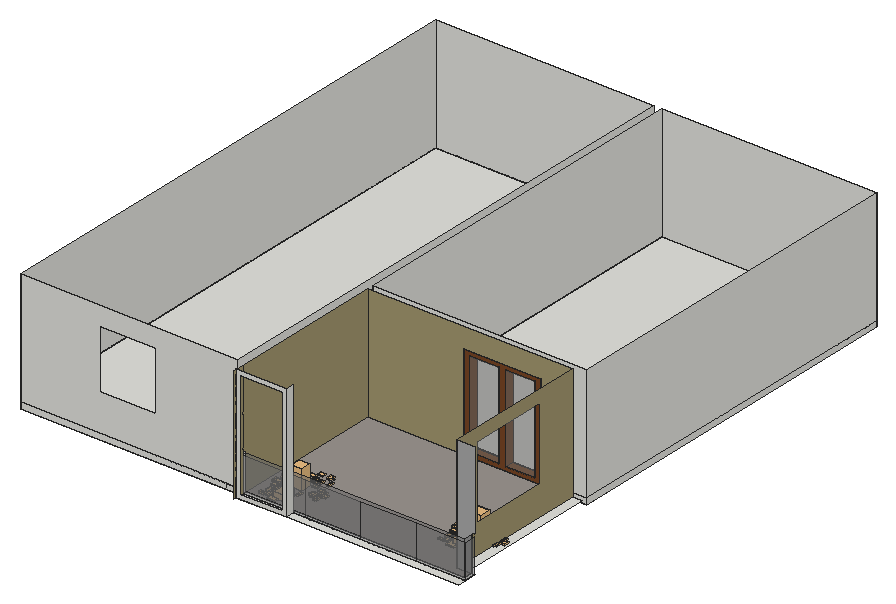
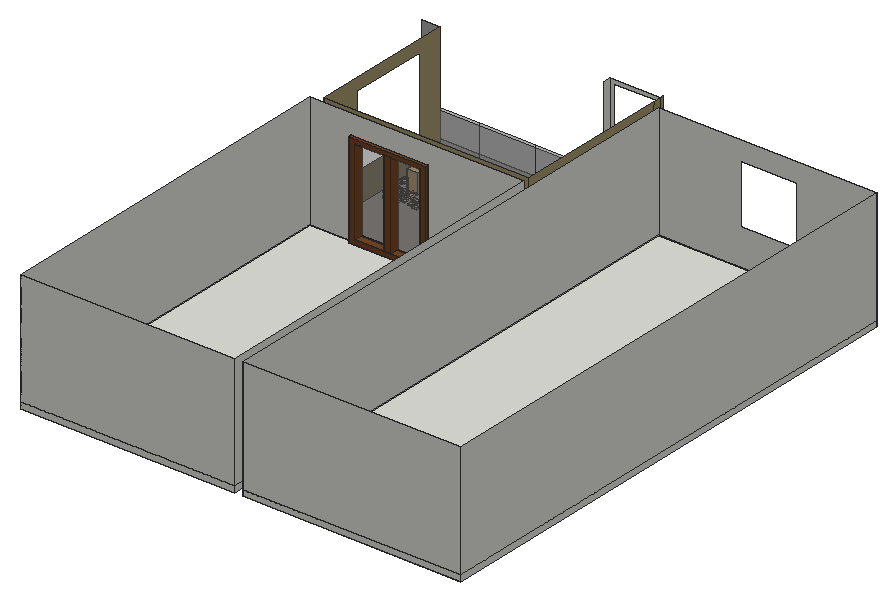
# SketchUp Ruby script. Lengths in inches.
U = 1.inch
M = Sketchup.active_model
def pt(a) = Geom::Point3d.new(a.map { |v| v * U })
def face(e, loops, mat)
  f = e.add_face(loops[0].map { |a| pt(a) })
  loops[1..].each { |l| e.add_face(l.map { |a| pt(a) }).erase! }
  f.material = f.back_material = mat if mat
  f
end
# faces: each face lists its corners as indices into pts; further lists are holes
def faces(e, pts, list, mat = nil) = list.each { |f| face(e, (f[0].is_a?(Array) ? f : [f]).map { |l| l.map { |i| pts[i] } }, mat) }
# xy, xz, yz: faces in a plane at the given z, y or x. An outline is a flat list of corners, or four numbers for a rectangle; further outlines are holes
def ring(l) = l.size == 4 ? [[l[0], l[1]], [l[2], l[1]], [l[2], l[3]], [l[0], l[3]]] : l.each_slice(2).to_a
def flat(e, list, mat, &to3) = list.each { |f| face(e, (f[0].is_a?(Array) ? f : [f]).map { |l| ring(l).map { |u, v| to3.(u, v) } }, mat) }
def xy(e, z, list, mat = nil) = flat(e, list, mat) { |x, y| [x, y, z] }
def xz(e, y, list, mat = nil) = flat(e, list, mat) { |x, z| [x, y, z] }
def yz(e, x, list, mat = nil) = flat(e, list, mat) { |y, z| [x, y, z] }
def lines(e, pts, list) = list.each { |a, b| e.add_line(pt(pts[a]), pt(pts[b])) }
# prism: a flat outline (further loops are holes) pulled along v
def prism(e, loops, v, mat = nil)
  f = face(e, loops, mat); d = Geom::Vector3d.new(v.map { |x| x * U })
  f.pushpull(f.normal.samedirection?(d) ? d.length : -d.length)
end
def box(e, o, s, mat = nil) = prism(e, [[o, [o[0] + s[0], o[1], o[2]], [o[0] + s[0], o[1] + s[1], o[2]], [o[0], o[1] + s[1], o[2]]]], [0, 0, s[2]], mat)
def at(x, y, z, deg = 0) = Geom::Transformation.translation(pt([x, y, z])) * Geom::Transformation.rotation(ORIGIN, Z_AXIS, deg.degrees)
def axes(o, x, y, z) = Geom::Transformation.new([*x, 0, *y, 0, *z, 0, *pt(o).to_a, 1])
def part(name) = M.definitions.add(name)
# library, detail: a bought-in or finely detailed component or shape, given as its bounding box
def library(name, o, s) = part(name).tap { |d| box(d.entities, o, s) }
def detail(e, o, s) = box(e.add_group.entities, o, s)
def put(e, d, t, mat = nil) = e.add_instance(d, t).tap { |i| i.material = mat if mat }
def group(e, t, mat = nil) = e.add_group.tap { |g| g.transformation = t; g.material = mat if mat }.entities
root = M.entities
M.materials.add("Bud_2").color = [160, 82, 113]
M.materials.add("Glass Realtime1").color = [156, 156, 156]
M.materials["Glass Realtime1"].alpha = 0.15
M.materials.add("Glass Red1").color = [0, 255, 255]
M.materials["Glass Red1"].alpha = 0.3
M.materials.add("Peony_Br1").color = [26, 30, 15]
M.materials.add("[Color M03]").color = [170, 170, 170]
M.materials.add("[Granite Tile]").color = [155, 148, 143]
M.materials.add("[Translucent Glass Gray]").color = [128, 128, 128]
M.materials["[Translucent Glass Gray]"].alpha = 0.5
M.materials.add("[Wood Lumber ButtJoined]").color = [164, 152, 112]
M.materials.add("[Wood Veneer 01]").color = [120, 70, 37]
c1 = part("Group\#1")
xy(c1.entities,0,[[0,0,48,9]],"[Wood Veneer 01]")
xy(c1.entities,3.71,[[3.71,0,21.93,9],[26.34,0,44.29,9]],"[Wood Veneer 01]")
xy(c1.entities,80.29,[[3.71,0,21.93,9],[26.34,0,44.29,9]],"[Wood Veneer 01]")
xy(c1.entities,84,[[0,0,48,9]],"[Wood Veneer 01]")
xz(c1.entities,0,[[3.71,3.71,21.93,80.29],[26.34,3.71,44.29,80.29]],"[Translucent Glass Gray]")
xz(c1.entities,0,[[[0,0,48,84],[3.71,3.71,21.93,80.29],[26.34,3.71,44.29,80.29]]],"[Wood Veneer 01]")
xz(c1.entities,9,[[[0,0,48,84],[3.71,3.71,44.29,80.29]],[21.93,3.71,26.34,80.29]],"[Wood Veneer 01]")
yz(c1.entities,0,[[0,0,9,84]],"[Wood Veneer 01]")
yz(c1.entities,3.71,[[0,3.71,9,80.29]],"[Wood Veneer 01]")
yz(c1.entities,21.93,[[0,3.71,9,80.29]],"[Wood Veneer 01]")
yz(c1.entities,26.34,[[0,3.71,9,80.29]],"[Wood Veneer 01]")
yz(c1.entities,44.29,[[0,3.71,9,80.29]],"[Wood Veneer 01]")
yz(c1.entities,48,[[0,0,9,84]],"[Wood Veneer 01]")
c2 = library("Group\#64",[-41.09,-203.71,-2.45],[72.23,68.1,8.96])
c3 = library("Group\#65",[-72.08,-328.41,-0.84],[78.06,90.26,14.33])
c4 = library("Group\#62",[-44.59,-71.91,-0.375],[108.06,108.06,265.92])
c5 = library("Group\#66",[-38.17,-273.34,-0.36],[93.61,85.68,37.86])
c6 = library("Group\#67",[-44.12,-281.8,-0.32],[111.26,106.83,75.57])
c7 = library("Group\#63",[-41.5,-68.73,2.45],[101.74,101.7,171.82])
xy(root,186,[[13.125,174.8125,241.5,718.875],[250.5,339.375,475.125,718.875]])
xy(root,192,[[250.5,161.01,303.24,169.32],[303.24,161.01,484.125,169.32],[250.5,169.32,250.5,173.51,480.43,173.51,480.43,182.19,484.125,182.19,484.125,169.32],[13.125,174.8125,241.5,718.875],[465.0625,182.19,475.125,333.375],
  [351.29,333.375,432.1,339.375],[250.5,339.375,475.125,718.875]])
xy(root,192,[[250.5,173.51,480.43,173.51,480.43,182.19,465.0625,182.19,465.0625,333.375,250.5,333.375]],"[Granite Tile]")
xz(root,161.01,[[[250.5,192,303.24,312.25],[254.52,196.02,299.22,308.23]]])
xz(root,169.32,[[250.5,192,303.24,228],[303.24,192,316.39,228],[316.39,192,374.26,228],[374.26,192,432.77,228],[432.77,192,484.125,228]],"[Translucent Glass Gray]")
xz(root,173.51,[[250.5,192,480.43,228]],"[Translucent Glass Gray]")
xz(root,174.8125,[[13.125,186,229,192],[229,186,241.5,192],[[13.125,192,241.5,312],[96.42,230.45,155.13,292.62]]])
xz(root,182.19,[[465.0625,192,480.43,192,480.43,230.3125,484.125,230.3125,484.125,312,465.0625,312]],"[Color M03]")
xz(root,333.375,[[250.5,192,351.29,192,351.29,291.4375,432.1,291.4375,432.1,192,465.0625,192,465.0625,312,250.5,312]],"[Wood Lumber ButtJoined]")
xz(root,339.375,[[250.5,186,351.29,192],[351.29,186,432.1,192],[432.1,186,445.8125,192],[445.8125,186,475.125,192],[250.5,192,250.5,312,475.125,312,475.125,192,432.1,192,432.1,291.4375,351.29,291.4375,351.29,192]])
xz(root,718.875,[[13.125,186,241.5,192],[250.5,186,475.125,192],[13.125,192,241.5,312],[250.5,192,475.125,312]])
yz(root,13.125,[[174.8125,186,718.875,192],[174.8125,192,718.875,312]])
yz(root,241.5,[[174.8125,186,718.875,192],[174.8125,192,718.875,312]])
yz(root,250.5,[[339.375,186,718.875,192],[169.32,192,173.51,228],[339.375,192,718.875,312]])
yz(root,250.5,[[157.82,192,161.01,312],[161.01,192,169.32,312],[173.51,192,333.375,192,333.375,312,169.32,312,169.32,230.3125,173.51,230.3125]],"[Wood Lumber ButtJoined]")
yz(root,303.24,[[161.01,192,169.32,312.25]])
yz(root,351.29,[[333.375,192,339.375,291.4375]])
yz(root,432.1,[[333.375,192,339.375,291.4375]])
yz(root,465.0625,[[[182.19,192,333.375,312],[207.39,223.41,290.14,299.35]]],"[Wood Lumber ButtJoined]")
yz(root,475.125,[[339.375,186,718.875,192],[339.375,192,718.875,312]])
yz(root,480.43,[[173.51,192,182.19,228]],"[Translucent Glass Gray]")
yz(root,484.125,[[169.32,192,182.19,228]],"[Translucent Glass Gray]")
p = [[279.06,209.92,192.1875],[279.16,209.92,192.1875],[279.16,210.03,192.1875],[441.92,241.33,192.1875],[442.03,241.33,192.1875],[442.03,241.44,192.1875]]
lines(root,p,[[0,1],[1,2],[2,0],[3,4],[4,5],[5,3]])
put(root,c1,axes([351.29,333.375,192],[1.68359,0,0],[0,1,0],[0,0,1.18378]))
put(root,c2,axes([279.06,209.92,192.1875],[0.1075,0,0],[0,0.1075,0],[0,0,0.0774]),"Peony_Br1")
put(root,c2,axes([441.92,241.33,192.1875],[0.1075,0,0],[0,0.1075,0],[0,0,0.0774]),"Peony_Br1")
g1 = group(root,at(279.06,209.92,192.1875),"Bud_2")
detail(g1,[-5.9,-14.63,-0.13],[5.36,2.04,0.85])
g2 = group(root,at(441.92,241.33,192.1875),"Bud_2")
detail(g2,[-5.9,-14.63,-0.13],[5.36,2.04,0.85])
g3 = group(root,at(279.06,209.92,192.1875),"Bud_2")
detail(g3,[20.81,-3.57,-0.13],[3.92,4.52,0.85])
g4 = group(root,at(441.92,241.33,192.1875),"Bud_2")
detail(g4,[20.81,-3.57,-0.13],[3.92,4.52,0.85])
g5 = group(root,at(279.06,209.92,192.1875),"Bud_2")
p = [[-13.21,22.51,0.21],[-13.11,22.36,0.08],[-13.21,23.11,-0.1],[-13.22,23.2,-0.04],[-15.51,18.89,0.15],[-14.6,19.57,0.01],
  [-13.87,20.48,0.33],[-15.4,18.86,-0.01],[-14.24,19.97,0.03],[-13.9,20.36,0.1],[-13.29,23.17,0.03],[-13.65,20.82,0.14],
  [-13.35,21.36,0.16],[-15.46,19.05,0.27],[-15.61,18.81,0.33],[-15.35,19.28,0.4],[-15.4,19.15,0.29],[-13.51,21.44,0.41],
  [-15.39,19.19,0.37],[-14.89,19.71,0.42],[-14.1,20.44,0.47],[-13.83,20.94,0.4375]]
faces(g5,p,[[0,1,2],[0,2,3],[4,5,6],[4,7,5],[8,6,5],[6,8,9],[3,10,0],[11,6,9],
  [6,11,12],[12,1,0],[4,13,14],[4,15,16],[13,4,16],[15,4,6],[6,12,17],[12,0,17],
  [15,18,16],[15,6,19],[6,20,19],[21,20,6],[6,17,21]],"Bud_2")
g6 = group(root,at(441.92,241.33,192.1875),"Bud_2")
p = [[-13.21,22.51,0.21],[-13.11,22.36,0.08],[-13.21,23.11,-0.1],[-13.22,23.2,-0.04],[-15.51,18.89,0.15],[-14.6,19.57,0.01],
  [-13.87,20.48,0.33],[-15.4,18.86,-0.01],[-14.24,19.97,0.03],[-13.9,20.36,0.1],[-13.29,23.17,0.03],[-13.65,20.82,0.14],
  [-13.35,21.36,0.16],[-15.46,19.05,0.27],[-15.61,18.81,0.33],[-15.35,19.28,0.4],[-15.4,19.15,0.29],[-13.51,21.44,0.41],
  [-15.39,19.19,0.37],[-14.89,19.71,0.42],[-14.1,20.44,0.47],[-13.83,20.94,0.4375]]
faces(g6,p,[[0,1,2],[0,2,3],[4,5,6],[4,7,5],[8,6,5],[6,8,9],[3,10,0],[11,6,9],
  [6,11,12],[12,1,0],[4,13,14],[4,15,16],[13,4,16],[15,4,6],[6,12,17],[12,0,17],
  [15,18,16],[15,6,19],[6,20,19],[21,20,6],[6,17,21]],"Bud_2")
g7 = group(root,at(279.06,209.92,192.1875),"Bud_2")
detail(g7,[2.23,12.49,-0.1],[2.04,5.3,0.86])
g8 = group(root,at(441.92,241.33,192.1875),"Bud_2")
detail(g8,[2.23,12.49,-0.1],[2.04,5.3,0.86])
g9 = group(root,at(279.06,209.92,192.1875),"Bud_2")
detail(g9,[-4.74,16.83,-0.09],[4.84,3.9,0.78])
g10 = group(root,at(441.92,241.33,192.1875),"Bud_2")
detail(g10,[-4.74,16.83,-0.09],[4.84,3.9,0.78])
g11 = group(root,at(279.06,209.92,192.1875),"Bud_2")
p = [[9.02,9.01,-0.02],[9.69,8.43,0],[9.61,8.46,-0.08],[8.9,9.11,0.18],[9.6,8.42,0.07],[7.97,9.7,0.3125],
  [7.95,9.77,0.01],[6.82,10.16,0.23],[7.27,9.95,0.02],[6.65,10.18,0.03],[4.65,10.31,-0.01],[4.16,10.26,0.24],
  [5.39,10.26,0.01],[4.48,10.27,0.1],[4.54,10.32,0.02],[4.35,10.29,0.13],[4.18,10.38,0.05],[7.27,9.87,0.37],
  [6.68,10.03,0.45],[6.07,10.0625,0.5],[5.45,10.14,0.5],[4.22,10.21,0.43]]
faces(g11,p,[[0,1,2],[0,3,4],[0,4,1],[5,0,6],[5,3,0],[7,5,6],[7,6,8],[8,9,7],
  [10,11,7],[10,7,12],[7,9,12],[11,10,13],[13,10,14],[11,15,16],[15,11,13],[7,17,5],
  [17,7,18],[7,19,18],[11,20,7],[11,21,20],[19,7,20]],"Bud_2")
g12 = group(root,at(441.92,241.33,192.1875),"Bud_2")
p = [[9.02,9.01,-0.02],[9.69,8.43,0],[9.61,8.46,-0.08],[8.9,9.11,0.18],[9.6,8.42,0.07],[7.97,9.7,0.3125],
  [7.95,9.77,0.01],[6.82,10.16,0.23],[7.27,9.95,0.02],[6.65,10.18,0.03],[4.65,10.31,-0.01],[4.16,10.26,0.24],
  [5.39,10.26,0.01],[4.48,10.27,0.1],[4.54,10.32,0.02],[4.35,10.29,0.13],[4.18,10.38,0.05],[7.27,9.87,0.37],
  [6.68,10.03,0.45],[6.07,10.0625,0.5],[5.45,10.14,0.5],[4.22,10.21,0.43]]
faces(g12,p,[[0,1,2],[0,3,4],[0,4,1],[5,0,6],[5,3,0],[7,5,6],[7,6,8],[8,9,7],
  [10,11,7],[10,7,12],[7,9,12],[11,10,13],[13,10,14],[11,15,16],[15,11,13],[7,17,5],
  [17,7,18],[7,19,18],[11,20,7],[11,21,20],[19,7,20]],"Bud_2")
g13 = group(root,at(279.06,209.92,192.1875),"Bud_2")
detail(g13,[-22.32,3.27,-0.07],[2.75,5.4,0.95])
g14 = group(root,at(441.92,241.33,192.1875),"Bud_2")
detail(g14,[-22.32,3.27,-0.07],[2.75,5.4,0.95])
g15 = group(root,at(279.06,209.92,192.1875),"Bud_2")
p = [[-7.58,-14.37,0.05],[-7.375,-14.31,-0.07],[-7.1,-13.11,0.05],[-7.67,-8.62,-0.0625],[-7.74,-8.53,-0.01],[-7.4375,-9.36,0.1],
  [-7.55,-9.5625,0.28],[-7.83,-8.61,0.04],[-7.77,-13.9,0.29],[-7.6875,-14.06,0.1875],[-7.15,-11.79,0.43],[-7.67,-14.1875,0.16],
  [-7.75,-14.37,0.23],[-7.02,-12.5,0.11],[-6.99,-11.9,0.22],[-7.39,-10.58,0.5],[-7.06,-10.58,0.3],[-7.75,-14.01,0.26],
  [-7.04,-11.29,0.26],[-7.63,-13.17,0.375],[-7.4,-11.95,0.52],[-7.42,-11.29,0.49]]
faces(g15,p,[[0,1,2],[3,4,5],[6,4,7],[6,5,4],[0,8,9],[8,0,10],[0,11,12],[11,0,9],
  [0,2,10],[13,10,2],[10,13,14],[15,5,6],[15,16,5],[9,8,17],[18,10,14],[8,10,19],
  [10,16,15],[10,18,16],[10,20,19],[10,21,20],[10,15,21]],"Bud_2")
g16 = group(root,at(441.92,241.33,192.1875),"Bud_2")
p = [[-7.58,-14.37,0.05],[-7.375,-14.31,-0.07],[-7.1,-13.11,0.05],[-7.67,-8.62,-0.0625],[-7.74,-8.53,-0.01],[-7.4375,-9.36,0.1],
  [-7.55,-9.5625,0.28],[-7.83,-8.61,0.04],[-7.77,-13.9,0.29],[-7.6875,-14.06,0.1875],[-7.15,-11.79,0.43],[-7.67,-14.1875,0.16],
  [-7.75,-14.37,0.23],[-7.02,-12.5,0.11],[-6.99,-11.9,0.22],[-7.39,-10.58,0.5],[-7.06,-10.58,0.3],[-7.75,-14.01,0.26],
  [-7.04,-11.29,0.26],[-7.63,-13.17,0.375],[-7.4,-11.95,0.52],[-7.42,-11.29,0.49]]
faces(g16,p,[[0,1,2],[3,4,5],[6,4,7],[6,5,4],[0,8,9],[8,0,10],[0,11,12],[11,0,9],
  [0,2,10],[13,10,2],[10,13,14],[15,5,6],[15,16,5],[9,8,17],[18,10,14],[8,10,19],
  [10,16,15],[10,18,16],[10,20,19],[10,21,20],[10,15,21]],"Bud_2")
g17 = group(root,at(279.06,209.92,192.1875),"Bud_2")
p = [[21.18,-5.17,0.05],[21.23,-4.96,-0.07],[20.34,-4.12,0.05],[16.16,-2.37,-0.0625],[16.05,-2.39,-0.01],[16.91,-2.54,0.1],
  [17.03,-2.74,0.28],[16.07,-2.5,0.04],[20.98,-5.16,0.16],[21.1,-5.3125,0.23],[19.17,-3.51,0.43],[20.68,-5.1,0.29],
  [20.86,-5.11,0.1875],[19.84,-3.75,0.11],[19.34,-3.42,0.22],[18,-3.11,0.5],[18.16,-2.83,0.3],[20.79,-5.13,0.26],
  [18.78,-3.16,0.26],[20.12,-4.62,0.375],[19.18,-3.81,0.52],[18.6,-3.49,0.49]]
faces(g17,p,[[0,1,2],[3,4,5],[6,4,7],[6,5,4],[0,8,9],[0,2,10],[11,0,10],[0,11,12],
  [8,0,12],[13,10,2],[10,13,14],[15,5,6],[15,16,5],[12,11,17],[18,10,14],[11,10,19],
  [10,16,15],[10,18,16],[10,20,19],[10,21,20],[10,15,21]],"Bud_2")
g18 = group(root,at(441.92,241.33,192.1875),"Bud_2")
p = [[21.18,-5.17,0.05],[21.23,-4.96,-0.07],[20.34,-4.12,0.05],[16.16,-2.37,-0.0625],[16.05,-2.39,-0.01],[16.91,-2.54,0.1],
  [17.03,-2.74,0.28],[16.07,-2.5,0.04],[20.98,-5.16,0.16],[21.1,-5.3125,0.23],[19.17,-3.51,0.43],[20.68,-5.1,0.29],
  [20.86,-5.11,0.1875],[19.84,-3.75,0.11],[19.34,-3.42,0.22],[18,-3.11,0.5],[18.16,-2.83,0.3],[20.79,-5.13,0.26],
  [18.78,-3.16,0.26],[20.12,-4.62,0.375],[19.18,-3.81,0.52],[18.6,-3.49,0.49]]
faces(g18,p,[[0,1,2],[3,4,5],[6,4,7],[6,5,4],[0,8,9],[0,2,10],[11,0,10],[0,11,12],
  [8,0,12],[13,10,2],[10,13,14],[15,5,6],[15,16,5],[12,11,17],[18,10,14],[11,10,19],
  [10,16,15],[10,18,16],[10,20,19],[10,21,20],[10,15,21]],"Bud_2")
put(root,c3,axes([279.06,209.92,192.1875],[0.1075,0,0],[0,0.1075,0],[0,0,0.0774]),"Peony_Br1")
put(root,c3,axes([441.92,241.33,192.1875],[0.1075,0,0],[0,0.1075,0],[0,0,0.0774]),"Peony_Br1")
g19 = group(root,at(279.06,209.92,192.1875),"Bud_2")
detail(g19,[-11.87,10.35,-0.0625],[4.93,4.51,0.74])
g20 = group(root,at(441.92,241.33,192.1875),"Bud_2")
detail(g20,[-11.87,10.35,-0.0625],[4.93,4.51,0.74])
g21 = group(root,at(279.06,209.92,192.1875),"Bud_2")
detail(g21,[-2.95,-13.39,-0.06],[2.25,5.14,0.71])
g22 = group(root,at(441.92,241.33,192.1875),"Bud_2")
detail(g22,[-2.95,-13.39,-0.06],[2.25,5.14,0.71])
g23 = group(root,at(279.06,209.92,192.1875),"Bud_2")
detail(g23,[17.98,-11.125,-0.05],[6.2,2.875,0.8])
g24 = group(root,at(441.92,241.33,192.1875),"Bud_2")
detail(g24,[17.98,-11.125,-0.05],[6.2,2.875,0.8])
g25 = group(root,at(279.06,209.92,192.1875),"Bud_2")
detail(g25,[-21.5,-9.1,-0.05],[6.35,4.98,1])
g26 = group(root,at(441.92,241.33,192.1875),"Bud_2")
detail(g26,[-21.5,-9.1,-0.05],[6.35,4.98,1])
g27 = group(root,at(279.06,209.92,192.1875),"Bud_2")
p = [[11.24,21.1,0.17],[12.16,22.02,-0.04],[13.25,22.87,0.28],[11.25,21.19,-0.01],[12.66,22.4,-0.03],[13.14,22.77,0.03],
  [13.71,23.03,0.08],[15.65,23.34,0.23],[15.47,23.45,0.08],[16.44,23.32,-0.03],[16.54,23.33,0.05],[14.35,23.34,0.11],
  [14.39,23.24,0.4],[16.48,23.28,0.12],[11.64,21.34,0.44],[11.51,21.26,0.32],[11.39,21.19,0.3],[11.24,21.1,0.38],
  [11.54,21.29,0.41],[12.21,21.83,0.44],[13.16,22.66,0.45],[13.77,22.91,0.43]]
faces(g27,p,[[0,1,2],[0,3,1],[4,2,1],[2,4,5],[6,2,5],[7,8,9],[7,9,10],[2,11,12],
  [2,6,11],[7,12,11],[7,11,8],[10,13,7],[0,14,15],[0,16,17],[16,0,15],[14,0,2],
  [15,14,18],[14,2,19],[2,20,19],[2,21,20],[12,21,2]],"Bud_2")
g28 = group(root,at(441.92,241.33,192.1875),"Bud_2")
p = [[11.24,21.1,0.17],[12.16,22.02,-0.04],[13.25,22.87,0.28],[11.25,21.19,-0.01],[12.66,22.4,-0.03],[13.14,22.77,0.03],
  [13.71,23.03,0.08],[15.65,23.34,0.23],[15.47,23.45,0.08],[16.44,23.32,-0.03],[16.54,23.33,0.05],[14.35,23.34,0.11],
  [14.39,23.24,0.4],[16.48,23.28,0.12],[11.64,21.34,0.44],[11.51,21.26,0.32],[11.39,21.19,0.3],[11.24,21.1,0.38],
  [11.54,21.29,0.41],[12.21,21.83,0.44],[13.16,22.66,0.45],[13.77,22.91,0.43]]
faces(g28,p,[[0,1,2],[0,3,1],[4,2,1],[2,4,5],[6,2,5],[7,8,9],[7,9,10],[2,11,12],
  [2,6,11],[7,12,11],[7,11,8],[10,13,7],[0,14,15],[0,16,17],[16,0,15],[14,0,2],
  [15,14,18],[14,2,19],[2,20,19],[2,21,20],[12,21,2]],"Bud_2")
g29 = group(root,at(279.06,209.92,192.1875),"Bud_2")
p = [[-8.66,14.35,0.55],[-8.67,14.46,0.49],[-10.8,15.02,-0.04],[-9.67,14.46,0.32],[-10.64,14.57,0.1],[-11.17,14.86,0],
  [-11.24,14.67,0.15],[-12.08,15.08,0.3],[-11.54,15.1875,0.16],[-13.82,15.57,0.05],[-13.57,15.88,0.04],[-13.74,16.03,0.03],
  [-13.43,15.85,0.0625],[-13.125,15.27,0.26],[-13.33,15.94,0.08],[-12.49,15.56,0.22],[-11.73,14.73,0.31],[-11.95,15.36,0.3],
  [-8.78,14.28,0.59],[-12.2,14.82,0.43],[-12.69,14.97,0.33]]
faces(g29,p,[[0,1,2],[2,3,0],[3,2,4],[5,4,2],[5,6,4],[7,6,5],[7,5,2],[7,2,8],
  [9,10,11],[9,12,10],[7,12,9],[13,7,9],[7,14,12],[7,15,14],[7,16,6],[7,17,15],
  [8,17,7],[18,0,3],[16,7,19],[7,20,19],[7,13,20]],"Bud_2")
g30 = group(root,at(441.92,241.33,192.1875),"Bud_2")
p = [[-8.66,14.35,0.55],[-8.67,14.46,0.49],[-10.8,15.02,-0.04],[-9.67,14.46,0.32],[-10.64,14.57,0.1],[-11.17,14.86,0],
  [-11.24,14.67,0.15],[-12.08,15.08,0.3],[-11.54,15.1875,0.16],[-13.82,15.57,0.05],[-13.57,15.88,0.04],[-13.74,16.03,0.03],
  [-13.43,15.85,0.0625],[-13.125,15.27,0.26],[-13.33,15.94,0.08],[-12.49,15.56,0.22],[-11.73,14.73,0.31],[-11.95,15.36,0.3],
  [-8.78,14.28,0.59],[-12.2,14.82,0.43],[-12.69,14.97,0.33]]
faces(g30,p,[[0,1,2],[2,3,0],[3,2,4],[5,4,2],[5,6,4],[7,6,5],[7,5,2],[7,2,8],
  [9,10,11],[9,12,10],[7,12,9],[13,7,9],[7,14,12],[7,15,14],[7,16,6],[7,17,15],
  [8,17,7],[18,0,3],[16,7,19],[7,20,19],[7,13,20]],"Bud_2")
g31 = group(root,at(279.06,209.92,192.1875),"Bud_2")
detail(g31,[-18.57,4.34,-0.04],[2.34,4.87,1.26])
g32 = group(root,at(441.92,241.33,192.1875),"Bud_2")
detail(g32,[-18.57,4.34,-0.04],[2.34,4.87,1.26])
g33 = group(root,at(279.06,209.92,192.1875),"Bud_2")
detail(g33,[-13.99,0.47,-0.04],[5.21,5.59,0.87])
g34 = group(root,at(441.92,241.33,192.1875),"Bud_2")
detail(g34,[-13.99,0.47,-0.04],[5.21,5.59,0.87])
g35 = group(root,at(279.06,209.92,192.1875),"Bud_2")
detail(g35,[-21.22,10.73,-0.04],[4.63,4.04,1.21])
g36 = group(root,at(441.92,241.33,192.1875),"Bud_2")
detail(g36,[-21.22,10.73,-0.04],[4.63,4.04,1.21])
g37 = group(root,at(279.06,209.92,192.1875),"Bud_2")
detail(g37,[17.42,0.48,-0.03],[4.12,3.84,0.71])
g38 = group(root,at(441.92,241.33,192.1875),"Bud_2")
detail(g38,[17.42,0.48,-0.03],[4.12,3.84,0.71])
g39 = group(root,at(279.06,209.92,192.1875),"Bud_2")
detail(g39,[7.79,-15.84,-0.03],[2.5,5.05,0.71])
g40 = group(root,at(441.92,241.33,192.1875),"Bud_2")
detail(g40,[7.79,-15.84,-0.03],[2.5,5.05,0.71])
g41 = group(root,at(279.06,209.92,192.1875),"Bud_2")
detail(g41,[-16.14,-25.87,-0.03],[1.25,5.39,1.93])
g42 = group(root,at(441.92,241.33,192.1875),"Bud_2")
detail(g42,[-16.14,-25.87,-0.03],[1.25,5.39,1.93])
g43 = group(root,at(279.06,209.92,192.1875),"Bud_2")
detail(g43,[-18.74,-31.57,-0.03],[5.12,2.12,1.39])
g44 = group(root,at(441.92,241.33,192.1875),"Bud_2")
detail(g44,[-18.74,-31.57,-0.03],[5.12,2.12,1.39])
put(root,c4,axes([279.06,209.92,192.1875],[0.1075,0,0],[0,0.1075,0],[0,0,0.0774]),"Glass Realtime1")
put(root,c4,axes([441.92,241.33,192.1875],[0.1075,0,0],[0,0.1075,0],[0,0,0.0774]),"Glass Realtime1")
put(root,c5,axes([279.06,209.92,192.1875],[0.1075,0,0],[0,0.1075,0],[0,0,0.0774]),"Peony_Br1")
put(root,c5,axes([441.92,241.33,192.1875],[0.1075,0,0],[0,0.1075,0],[0,0,0.0774]),"Peony_Br1")
g45 = group(root,at(279.06,209.92,192.1875),"Bud_2")
p = [[-4.24,-9.44,0.05],[-4.38,-10.24,0.125],[-4.45,-10.28,0.05],[-4.41,-10.21,-0.03],[-4.16,-9.26,0.25],[-3.78,-8.2,0.1],
  [-3.73,-8.28,0.39],[-2.99,-7.32,0.3],[-2.83,-7.2,0.1],[-1.74,-6.58,0.03],[-1.1,-6.2,-0.01],[-0.625,-6.03,0.23],
  [-0.92,-6.16,0.1],[-1,-6.14,0.02],[-0.82,-6.09,0.12],[-0.71,-5.93,0.04],[-3.27,-7.7,0.09],[-1.7,-6.72,0.52],
  [-0.64,-6.12,0.41],[-3.21,-7.78,0.44],[-2.76,-7.37,0.51],[-2.22,-7.07,0.54]]
faces(g45,p,[[0,1,2],[2,3,0],[0,4,1],[5,6,0],[6,4,0],[7,8,9],[10,7,9],[10,11,7],
  [11,10,12],[12,10,13],[11,14,15],[7,6,5],[7,5,16],[7,16,8],[14,11,12],[11,17,7],
  [11,18,17],[7,19,6],[19,7,20],[7,21,20],[21,7,17]],"Bud_2")
g46 = group(root,at(441.92,241.33,192.1875),"Bud_2")
p = [[-4.24,-9.44,0.05],[-4.38,-10.24,0.125],[-4.45,-10.28,0.05],[-4.41,-10.21,-0.03],[-4.16,-9.26,0.25],[-3.78,-8.2,0.1],
  [-3.73,-8.28,0.39],[-2.99,-7.32,0.3],[-2.83,-7.2,0.1],[-1.74,-6.58,0.03],[-1.1,-6.2,-0.01],[-0.625,-6.03,0.23],
  [-0.92,-6.16,0.1],[-1,-6.14,0.02],[-0.82,-6.09,0.12],[-0.71,-5.93,0.04],[-3.27,-7.7,0.09],[-1.7,-6.72,0.52],
  [-0.64,-6.12,0.41],[-3.21,-7.78,0.44],[-2.76,-7.37,0.51],[-2.22,-7.07,0.54]]
faces(g46,p,[[0,1,2],[2,3,0],[0,4,1],[5,6,0],[6,4,0],[7,8,9],[10,7,9],[10,11,7],
  [11,10,12],[12,10,13],[11,14,15],[7,6,5],[7,5,16],[7,16,8],[14,11,12],[11,17,7],
  [11,18,17],[7,19,6],[19,7,20],[7,21,20],[21,7,17]],"Bud_2")
put(root,c6,axes([279.06,209.92,192.1875],[0.1075,0,0],[0,0.1075,0],[0,0,0.0774]),"Bud_2")
put(root,c6,axes([441.92,241.33,192.1875],[0.1075,0,0],[0,0.1075,0],[0,0,0.0774]),"Bud_2")
g47 = group(root,at(279.06,209.92,192.1875),"Bud_2")
detail(g47,[-24.68,16.18,-0.02],[5.31,2.02,0.74])
g48 = group(root,at(441.92,241.33,192.1875),"Bud_2")
detail(g48,[-24.68,16.18,-0.02],[5.31,2.02,0.74])
g49 = group(root,at(279.06,209.92,192.1875),"Bud_2")
detail(g49,[-13.74,-19.43,-0.02],[3.5,5.54,0.81])
g50 = group(root,at(441.92,241.33,192.1875),"Bud_2")
detail(g50,[-13.74,-19.43,-0.02],[3.5,5.54,0.81])
g51 = group(root,at(279.06,209.92,192.1875),"Bud_2")
detail(g51,[22.58,-3.19,-0.02],[4.21,5.66,1.15])
g52 = group(root,at(441.92,241.33,192.1875),"Bud_2")
detail(g52,[22.58,-3.19,-0.02],[4.21,5.66,1.15])
g53 = group(root,at(279.06,209.92,192.1875),"Bud_2")
detail(g53,[-13.66,-30.82,-0.01],[3.6,5.41,0.92])
g54 = group(root,at(441.92,241.33,192.1875),"Bud_2")
detail(g54,[-13.66,-30.82,-0.01],[3.6,5.41,0.92])
g55 = group(root,at(279.06,209.92,192.1875),"Bud_2")
detail(g55,[-19.59,-15.02,-0.01],[6.1,4.3,1.1])
g56 = group(root,at(441.92,241.33,192.1875),"Bud_2")
detail(g56,[-19.59,-15.02,-0.01],[6.1,4.3,1.1])
g57 = group(root,at(279.06,209.92,192.1875),"Bud_2")
detail(g57,[-22.52,-9.47,-0.01],[1.45,5.49,1.23])
g58 = group(root,at(441.92,241.33,192.1875),"Bud_2")
detail(g58,[-22.52,-9.47,-0.01],[1.45,5.49,1.23])
g59 = group(root,at(279.06,209.92,192.1875),"Bud_2")
detail(g59,[26.73,-5.87,-0.01],[3.91,4.56,1.35])
g60 = group(root,at(441.92,241.33,192.1875),"Bud_2")
detail(g60,[26.73,-5.87,-0.01],[3.91,4.56,1.35])
g61 = group(root,at(279.06,209.92,192.1875),"Bud_2")
detail(g61,[-19.41,20.4,0],[5.31,3.52,1.58])
g62 = group(root,at(441.92,241.33,192.1875),"Bud_2")
detail(g62,[-19.41,20.4,0],[5.31,3.52,1.58])
g63 = group(root,at(279.06,209.92,192.1875),"Bud_2")
detail(g63,[-4.3,7.33,0],[4.16,5.19,2.05])
g64 = group(root,at(441.92,241.33,192.1875),"Bud_2")
detail(g64,[-4.3,7.33,0],[4.16,5.19,2.05])
g65 = group(root,at(279.06,209.92,192.1875),"Bud_2")
p = [[-10.97,-5.54,0.2],[-10.36,-6.01,0.01],[-10.41,-6.15,0.03],[-10.51,-6.13,0.01],[-10.83,-5.31,0.28],[-12.14,-3.64,0.17],
  [-12.32,-3.27,0],[-12.11,-3.07,0.08],[-12.6875,-2.8125,0.02],[-11.71,-3.33,0.17],[-11.85,-2.88,0.04],[-13.33,-2.11,0.04],
  [-13.28,-2,0.09],[-12.16,-2.45,0.09],[-11.9,-4.35,0.4],[-11.83,-3.95,0.41],[-11.61,-3.8125,0.33],[-13.14,-1.5625,0.18],
  [-12.58,-2.12,0.07],[-13.36,-1.875,0.1],[-13.54,-1.75,0.0625],[-11.38,-4.37,0.4]]
faces(g65,p,[[0,1,2],[0,2,3],[0,4,1],[5,6,7],[7,6,8],[9,7,10],[7,8,11],[7,11,12],
  [7,13,10],[7,14,5],[7,15,14],[7,16,15],[7,9,16],[7,12,17],[18,7,17],[7,18,13],
  [17,12,19],[17,19,20],[0,14,21],[0,21,4],[15,16,21],[15,21,14]],"Bud_2")
g66 = group(root,at(441.92,241.33,192.1875),"Bud_2")
p = [[-10.97,-5.54,0.2],[-10.36,-6.01,0.01],[-10.41,-6.15,0.03],[-10.51,-6.13,0.01],[-10.83,-5.31,0.28],[-12.14,-3.64,0.17],
  [-12.32,-3.27,0],[-12.11,-3.07,0.08],[-12.6875,-2.8125,0.02],[-11.71,-3.33,0.17],[-11.85,-2.88,0.04],[-13.33,-2.11,0.04],
  [-13.28,-2,0.09],[-12.16,-2.45,0.09],[-11.9,-4.35,0.4],[-11.83,-3.95,0.41],[-11.61,-3.8125,0.33],[-13.14,-1.5625,0.18],
  [-12.58,-2.12,0.07],[-13.36,-1.875,0.1],[-13.54,-1.75,0.0625],[-11.38,-4.37,0.4]]
faces(g66,p,[[0,1,2],[0,2,3],[0,4,1],[5,6,7],[7,6,8],[9,7,10],[7,8,11],[7,11,12],
  [7,13,10],[7,14,5],[7,15,14],[7,16,15],[7,9,16],[7,12,17],[18,7,17],[7,18,13],
  [17,12,19],[17,19,20],[0,14,21],[0,21,4],[15,16,21],[15,21,14]],"Bud_2")
g67 = group(root,at(279.06,209.92,192.1875),"Bud_2")
detail(g67,[1.125,8.26,0.01],[3.04,6.12,1.04])
g68 = group(root,at(441.92,241.33,192.1875),"Bud_2")
detail(g68,[1.125,8.26,0.01],[3.04,6.12,1.04])
g69 = group(root,at(279.06,209.92,192.1875),"Bud_2")
detail(g69,[-12.13,18.29,0.02],[3.6,4.1,0.96])
g70 = group(root,at(441.92,241.33,192.1875),"Bud_2")
detail(g70,[-12.13,18.29,0.02],[3.6,4.1,0.96])
g71 = group(root,at(279.06,209.92,192.1875),"Bud_2")
detail(g71,[22.65,-11.72,0.02],[3.9,5.43,0.77])
g72 = group(root,at(441.92,241.33,192.1875),"Bud_2")
detail(g72,[22.65,-11.72,0.02],[3.9,5.43,0.77])
g73 = group(root,at(279.06,209.92,192.1875),"Bud_2")
detail(g73,[-15.2,-12.1875,0.02],[2.2,6.61,1.09])
g74 = group(root,at(441.92,241.33,192.1875),"Bud_2")
detail(g74,[-15.2,-12.1875,0.02],[2.2,6.61,1.09])
g75 = group(root,at(279.06,209.92,192.1875),"Bud_2")
detail(g75,[-0.09,22.24,0.02],[5.12,4.26,0.9])
g76 = group(root,at(441.92,241.33,192.1875),"Bud_2")
detail(g76,[-0.09,22.24,0.02],[5.12,4.26,0.9])
g77 = group(root,at(279.06,209.92,192.1875),"Bud_2")
detail(g77,[-10.69,-22.22,0.03],[4.02,5.24,0.76])
g78 = group(root,at(441.92,241.33,192.1875),"Bud_2")
detail(g78,[-10.69,-22.22,0.03],[4.02,5.24,0.76])
g79 = group(root,at(279.06,209.92,192.1875),"Bud_2")
detail(g79,[8.89,3.86,0.03],[5.69,2.76,0.8])
g80 = group(root,at(441.92,241.33,192.1875),"Bud_2")
detail(g80,[8.89,3.86,0.03],[5.69,2.76,0.8])
g81 = group(root,at(279.06,209.92,192.1875),"Bud_2")
detail(g81,[-12.52,-14.06,0.03],[1.54,6.14,1.21])
g82 = group(root,at(441.92,241.33,192.1875),"Bud_2")
detail(g82,[-12.52,-14.06,0.03],[1.54,6.14,1.21])
g83 = group(root,at(279.06,209.92,192.1875),"Bud_2")
detail(g83,[-13.21,-21.09,0.04],[5.17,2.79,1.07])
g84 = group(root,at(441.92,241.33,192.1875),"Bud_2")
detail(g84,[-13.21,-21.09,0.04],[5.17,2.79,1.07])
g85 = group(root,at(279.06,209.92,192.1875),"Bud_2")
detail(g85,[17.64,11.49,0.05],[2.95,6.5,1.15])
g86 = group(root,at(441.92,241.33,192.1875),"Bud_2")
detail(g86,[17.64,11.49,0.05],[2.95,6.5,1.15])
g87 = group(root,at(279.06,209.92,192.1875),"Bud_2")
p = [[-2.97,6.74,0.27],[-1.6875,7.34,0.11],[-1.68,7.7,0.05],[-2.32,7.41,0.18],[-1.42,7.48,0.2],[-4.82,5.01,0.41],
  [-3.43,5.75,0.15],[-3.9,5.83,0.125],[-3.57,6.25,0.1],[-3.37,6.63,0.2],[-1.69,7.24,0.24],[-5.0625,4.64,0.61],
  [-3.1,6.27,0.27],[-3.14,6.99,0.26],[-2.75,7.24,0.18],[-2.42,6.84,0.3125],[-2.86,6.57,0.37],[-5.17,4.66,0.57],
  [-5.18,4.76,0.57]]
faces(g87,p,[[0,1,2],[3,0,2],[2,1,4],[5,6,7],[7,6,8],[0,8,6],[0,9,8],[0,10,1],
  [5,11,6],[0,6,12],[0,13,9],[13,0,14],[0,3,14],[0,15,10],[12,16,0],[0,16,15],
  [17,11,5],[5,18,17]],"Bud_2")
g88 = group(root,at(441.92,241.33,192.1875),"Bud_2")
p = [[-2.97,6.74,0.27],[-1.6875,7.34,0.11],[-1.68,7.7,0.05],[-2.32,7.41,0.18],[-1.42,7.48,0.2],[-4.82,5.01,0.41],
  [-3.43,5.75,0.15],[-3.9,5.83,0.125],[-3.57,6.25,0.1],[-3.37,6.63,0.2],[-1.69,7.24,0.24],[-5.0625,4.64,0.61],
  [-3.1,6.27,0.27],[-3.14,6.99,0.26],[-2.75,7.24,0.18],[-2.42,6.84,0.3125],[-2.86,6.57,0.37],[-5.17,4.66,0.57],
  [-5.18,4.76,0.57]]
faces(g88,p,[[0,1,2],[3,0,2],[2,1,4],[5,6,7],[7,6,8],[0,8,6],[0,9,8],[0,10,1],
  [5,11,6],[0,6,12],[0,13,9],[13,0,14],[0,3,14],[0,15,10],[12,16,0],[0,16,15],
  [17,11,5],[5,18,17]],"Bud_2")
g89 = group(root,at(279.06,209.92,192.1875),"Bud_2")
detail(g89,[-8.74,-4.75,0.05],[4.17,5.12,1.35])
g90 = group(root,at(441.92,241.33,192.1875),"Bud_2")
detail(g90,[-8.74,-4.75,0.05],[4.17,5.12,1.35])
g91 = group(root,at(279.06,209.92,192.1875),"Bud_2")
detail(g91,[-20.39,-0.9,0.05],[5.2,3.43,0.77])
g92 = group(root,at(441.92,241.33,192.1875),"Bud_2")
detail(g92,[-20.39,-0.9,0.05],[5.2,3.43,0.77])
g93 = group(root,at(279.06,209.92,192.1875),"Bud_2")
detail(g93,[10.88,20.74,0.07],[3.28,5.49,1.47])
g94 = group(root,at(441.92,241.33,192.1875),"Bud_2")
detail(g94,[10.88,20.74,0.07],[3.28,5.49,1.47])
g95 = group(root,at(279.06,209.92,192.1875),"Bud_2")
detail(g95,[8.59,11,0.07],[4.02,5.23,0.77])
g96 = group(root,at(441.92,241.33,192.1875),"Bud_2")
detail(g96,[8.59,11,0.07],[4.02,5.23,0.77])
g97 = group(root,at(279.06,209.92,192.1875),"Bud_2")
detail(g97,[15.32,-8.5625,0.08],[4.62,4.26,1.2])
g98 = group(root,at(441.92,241.33,192.1875),"Bud_2")
detail(g98,[15.32,-8.5625,0.08],[4.62,4.26,1.2])
g99 = group(root,at(279.06,209.92,192.1875),"Bud_2")
detail(g99,[6.07,12.125,0.08],[5.17,2.8,1.08])
g100 = group(root,at(441.92,241.33,192.1875),"Bud_2")
detail(g100,[6.07,12.125,0.08],[5.17,2.8,1.08])
g101 = group(root,at(279.06,209.92,192.1875),"Bud_2")
detail(g101,[23.75,-13.39,0.08],[1.48,5.6,1.08])
g102 = group(root,at(441.92,241.33,192.1875),"Bud_2")
detail(g102,[23.75,-13.39,0.08],[1.48,5.6,1.08])
g103 = group(root,at(279.06,209.92,192.1875),"Bud_2")
detail(g103,[2.35,3.24,0.09],[2.13,4.65,0.71])
g104 = group(root,at(441.92,241.33,192.1875),"Bud_2")
detail(g104,[2.35,3.24,0.09],[2.13,4.65,0.71])
g105 = group(root,at(279.06,209.92,192.1875),"Bud_2")
detail(g105,[-8.54,-9.74,0.1],[3,4.72,0.95])
g106 = group(root,at(441.92,241.33,192.1875),"Bud_2")
detail(g106,[-8.54,-9.74,0.1],[3,4.72,0.95])
g107 = group(root,at(279.06,209.92,192.1875),"Bud_2")
detail(g107,[2.83,8.0625,0.1],[5.74,2.09,1.16])
g108 = group(root,at(441.92,241.33,192.1875),"Bud_2")
detail(g108,[2.83,8.0625,0.1],[5.74,2.09,1.16])
g109 = group(root,at(279.06,209.92,192.1875),"Bud_2")
detail(g109,[-2.7,3.58,0.12],[3.2,4.58,1.25])
g110 = group(root,at(441.92,241.33,192.1875),"Bud_2")
detail(g110,[-2.7,3.58,0.12],[3.2,4.58,1.25])
put(root,c7,axes([279.06,209.92,192.1875],[0.1075,0,0],[0,0.1075,0],[0,0,0.0774]),"Glass Red1")
put(root,c7,axes([441.92,241.33,192.1875],[0.1075,0,0],[0,0.1075,0],[0,0,0.0774]),"Glass Red1")
